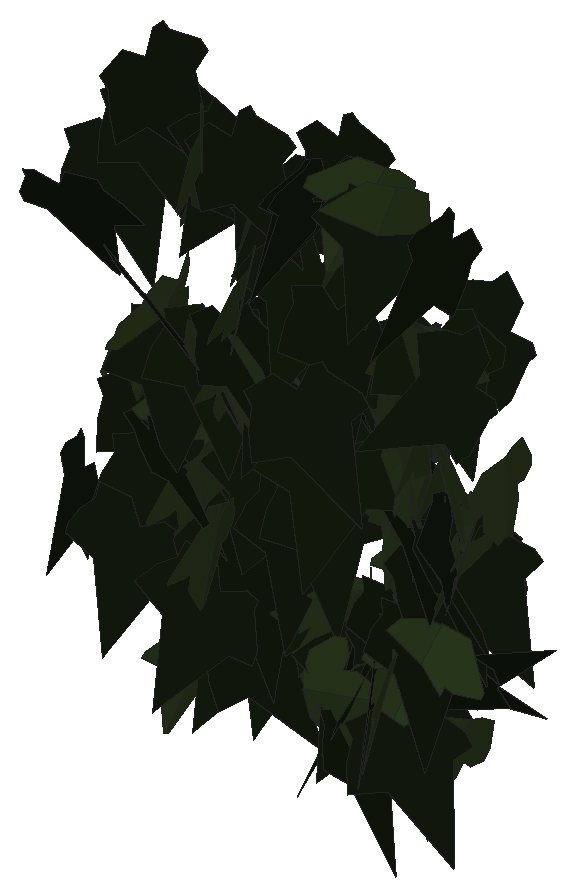
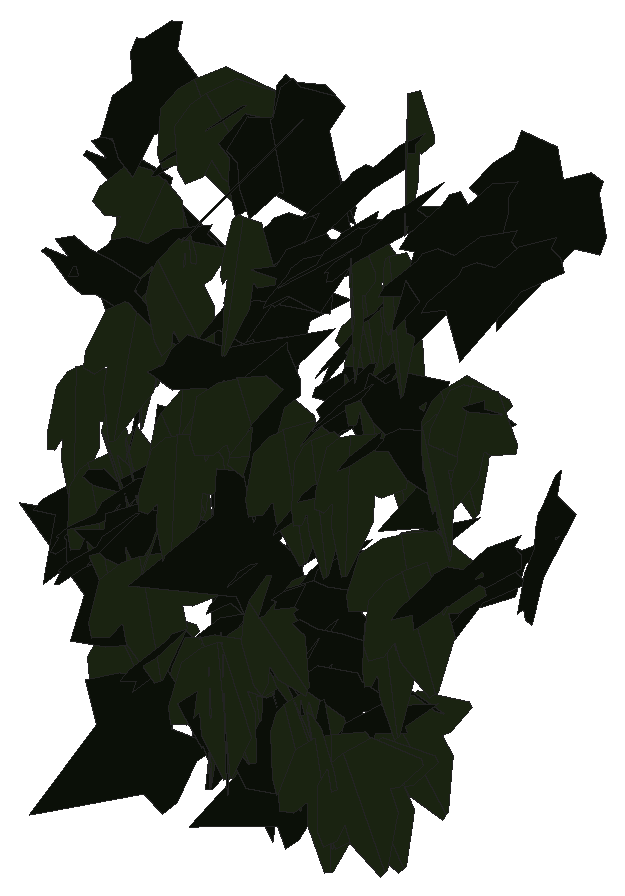
# SketchUp Ruby script. Lengths in inches.
U = 1.inch
M = Sketchup.active_model
def pt(a) = Geom::Point3d.new(a.map { |v| v * U })
def face(e, loops, mat)
  f = e.add_face(loops[0].map { |a| pt(a) })
  loops[1..].each { |l| e.add_face(l.map { |a| pt(a) }).erase! }
  f.material = f.back_material = mat if mat
  f
end
# faces: each face lists its corners as indices into pts; further lists are holes
def faces(e, pts, list, mat = nil) = list.each { |f| face(e, (f[0].is_a?(Array) ? f : [f]).map { |l| l.map { |i| pts[i] } }, mat) }
# xy, xz, yz: faces in a plane at the given z, y or x. An outline is a flat list of corners, or four numbers for a rectangle; further outlines are holes
def ring(l) = l.size == 4 ? [[l[0], l[1]], [l[2], l[1]], [l[2], l[3]], [l[0], l[3]]] : l.each_slice(2).to_a
def flat(e, list, mat, &to3) = list.each { |f| face(e, (f[0].is_a?(Array) ? f : [f]).map { |l| ring(l).map { |u, v| to3.(u, v) } }, mat) }
def xy(e, z, list, mat = nil) = flat(e, list, mat) { |x, y| [x, y, z] }
def xz(e, y, list, mat = nil) = flat(e, list, mat) { |x, z| [x, y, z] }
def yz(e, x, list, mat = nil) = flat(e, list, mat) { |y, z| [x, y, z] }
def lines(e, pts, list) = list.each { |a, b| e.add_line(pt(pts[a]), pt(pts[b])) }
# prism: a flat outline (further loops are holes) pulled along v
def prism(e, loops, v, mat = nil)
  f = face(e, loops, mat); d = Geom::Vector3d.new(v.map { |x| x * U })
  f.pushpull(f.normal.samedirection?(d) ? d.length : -d.length)
end
def box(e, o, s, mat = nil) = prism(e, [[o, [o[0] + s[0], o[1], o[2]], [o[0] + s[0], o[1] + s[1], o[2]], [o[0], o[1] + s[1], o[2]]]], [0, 0, s[2]], mat)
def at(x, y, z, deg = 0) = Geom::Transformation.translation(pt([x, y, z])) * Geom::Transformation.rotation(ORIGIN, Z_AXIS, deg.degrees)
def axes(o, x, y, z) = Geom::Transformation.new([*x, 0, *y, 0, *z, 0, *pt(o).to_a, 1])
def part(name) = M.definitions.add(name)
# library, detail: a bought-in or finely detailed component or shape, given as its bounding box
def library(name, o, s) = part(name).tap { |d| box(d.entities, o, s) }
def detail(e, o, s) = box(e.add_group.entities, o, s)
def put(e, d, t, mat = nil) = e.add_instance(d, t).tap { |i| i.material = mat if mat }
def group(e, t, mat = nil) = e.add_group.tap { |g| g.transformation = t; g.material = mat if mat }.entities
root = M.entities
M.materials.add("efeu1").color = [18, 25, 13]
M.materials.add("efeu2").color = [43, 57, 29]
c1 = part("ivyleaf_9")
p = [[1.54,2.16,1.25],[1.36,2.04,1.19],[-0.21,0.99,0.68],[-0.71,1.11,0.82],[-0.85,0.86,0.67],[-0.8,0.17,0.21],
  [-0.9,-0.01,0.1],[-0.67,-0.16,-0.02],[-0.08,-0.08,-0.05],[-0.03,-0.6,-0.4],[0.65,-0.88,-0.66],[0.83,-0.6,-0.49],
  [1.29,-0.42,-0.43],[1.8125,-0.07,-0.26],[1.21,0.44,0.15]]
faces(c1.entities,p,[[0,1,2,3,4,5,6,7,8,9,10,11,12,13,14]],"efeu1")
c2 = part("ivyleaf_10")
p = [[0,0.5,-0.03],[-0.0625,2.02,-0.43],[-0.19,2.01,-0.46],[-0.54,1.05,-0.29],[-0.52,0.625,-0.18],[-0.83,0.76,-0.28],
  [-1.16,0.64,-0.33],[-1.15,0.33,-0.24],[-0.77,-0.39,0.02],[-0.3,-0.51,0.16],[0.04,-0.48,0.23],[-0.02,2.01,-0.4375],
  [-0.06,2.01,-0.43],[0.04,-0.49,0.23],[0.67,-0.49,0.14],[1.38,0.36,-0.2],[1.375,0.51,-0.24],[0.81,0.65,-0.19],
  [0.62,0.59,-0.15],[0.6,1.09,-0.28],[0.5,1.23,-0.31]]
faces(c2.entities,p,[[0,1,2,3,4,5,6,7,8,9,10],[11,12,0,13,14,15,16,17,18,19,20]],"efeu2")
put(root,c1,axes([21.94,221.7,247.83],[-0.00718,-0.45611,-0.20472],[0.00835,0.2046,-0.45615],[0.49988,-0.00997,0.00468]))
put(root,c1,axes([21.98,222.09,248.62],[0.12472,-0.32873,-0.35551],[-0.11519,0.33643,-0.35149],[0.47029,0.16958,0.00819]))
put(root,c1,axes([21.98,222.13,244.82],[0.06592,-0.45564,-0.19506],[-0.00933,0.1956,-0.46006],[0.49555,0.06429,0.01728]))
put(root,c1,axes([22.02,222.2,248.14],[-0.002,-0.44065,-0.23628],[0.02599,0.23587,-0.4401],[0.49932,-0.01404,0.02196]))
put(root,c2,axes([22.24,222.24,246.03],[0.20254,-0.45532,-0.04074],[-0.00639,0.04173,-0.49821],[0.4571,0.20233,0.01109]))
put(root,c1,axes([22.11,220.87,244.48],[0.0514,-0.1225,-0.48203],[0.39843,-0.2799,0.11362],[-0.29768,-0.39579,0.06885]))
put(root,c1,axes([22.26,220.36,248.03],[0.43986,0.19109,-0.14144],[-0.12527,-0.06654,-0.47946],[-0.20207,0.45723,-0.01067]))
put(root,c2,axes([22.37,221.54,246.09],[-0.05994,-0.43878,-0.23212],[0.06327,0.22515,-0.44193],[0.49235,-0.08235,0.02853]))
put(root,c2,axes([22.43,222.34,244.48],[-0.20804,-0.43866,0.11957],[0.00303,-0.13282,-0.48203],[0.45465,-0.19984,0.05793]))
put(root,c2,axes([22.47,221.68,246.08],[-0.01427,-0.49342,0.07959],[0.00788,-0.07984,-0.49352],[0.49973,-0.01283,0.01005]))
put(root,c2,axes([22.53,222.3,244.82],[-0.35573,-0.34113,0.08416],[0.01746,-0.13678,-0.48061],[0.35093,-0.339,0.10922]))
put(root,c2,axes([22.67,222.24,247.66],[0.13927,-0.44991,-0.16789],[-0.04136,0.16292,-0.4709],[0.47843,0.14505,0.00817]))
put(root,c1,axes([22.47,221.78,244.32],[-0.09242,-0.47478,-0.12667],[0.04032,0.12113,-0.48343],[0.48973,-0.09957,0.0159]))
put(root,c2,axes([22.8125,222.1875,243.95],[0.04057,-0.49503,-0.05741],[0.00034,0.05762,-0.49667],[0.49835,0.04026,0.00501]))
put(root,c1,axes([22.7,221.02,243.94],[-0.10273,-0.46976,0.13699],[0.00798,-0.14157,-0.47947],[0.48927,-0.09633,0.03658]))
put(root,c1,axes([22.72,221.72,245.86],[-0.14691,-0.46907,-0.09159],[0.03101,0.08626,-0.49153],[0.47692,-0.1501,0.00375]))
put(root,c2,axes([22.93,222.54,242.49],[-0.10601,-0.47011,0.13326],[-0.00024,-0.13631,-0.48106],[0.48863,-0.10206,0.02867]))
put(root,c2,axes([22.92,221.68,244.43],[-0.0495,-0.47632,-0.14378],[0.03239,0.1411,-0.47858],[0.49649,-0.05669,0.01688]))
put(root,c2,axes([22.99,222.29,242.35],[-0.13086,-0.44973,0.17498],[-0.01304,-0.17794,-0.46709],[0.48239,-0.12681,0.03484]))
put(root,c2,axes([23.04,222.43,245.72],[-0.05034,-0.47661,-0.14251],[0.0096,0.14228,-0.47923],[0.49737,-0.05098,-0.00517]))
put(root,c2,axes([23.06,221.63,242.52],[-0.08309,-0.44521,0.21185],[0.00959,-0.21626,-0.45071],[0.49295,-0.07084,0.04448]))
put(root,c2,axes([23.19,222.53,242.5625],[-0.22687,-0.44358,-0.04205],[0.02165,0.03615,-0.49822],[0.44504,-0.22788,0.0028]))
put(root,c1,axes([22.86,221.06,245.08],[0.3603,-0.34484,0.0357],[0.03065,-0.0196,-0.49867],[0.34532,0.36153,0.00701]))
put(root,c1,axes([23.11,222.16,247.91],[-0.15095,-0.40278,0.25491],[-0.02749,-0.25959,-0.42645],[0.47588,-0.14276,0.05622]))
put(root,c2,axes([23.3125,222.59,245.65],[0.03476,-0.49595,-0.05316],[0.00722,0.05379,-0.49705],[0.49874,0.03379,0.0109]))
put(root,c1,axes([23.27,222.25,242.69],[-0.23801,-0.4244,0.11505],[-0.0315,-0.11403,-0.4858],[0.43859,-0.2385,0.02754]))
put(root,c1,axes([23.14,222.59,245.61],[0.04574,-0.49787,-0.00559],[-0.00178,0.00545,-0.49997],[0.4979,0.04575,-0.00127]))
put(root,c2,axes([23.36,222.54,242.77],[0.33224,-0.35276,-0.12319],[-0.04442,0.12638,-0.48172],[0.371,0.33104,0.05264]))
put(root,c1,axes([23.25,221.66,246.13],[-0.24943,-0.34197,-0.26616],[0.18372,0.19468,-0.42231],[0.39247,-0.30847,0.02854]))
put(root,c2,axes([23.41,221.08,248.6],[0.19754,-0.42153,-0.18247],[0.00708,0.2014,-0.45759],[0.45927,0.1782,0.08554]))
put(root,c2,axes([23.43,221.9,247.39],[0.22939,-0.42739,-0.12134],[0.01425,0.14356,-0.47874],[0.44405,0.21617,0.07804]))
put(root,c1,axes([23.09,220.61,247],[0.16255,-0.31502,0.35262],[0.24397,-0.26354,-0.34789],[0.40504,0.28516,0.06803]))
put(root,c1,axes([23.5,222.36,244.3],[-0.21717,-0.42753,0.14161],[-0.02373,-0.14614,-0.47758],[0.44975,-0.21415,0.04319]))
put(root,c1,axes([23.4375,221.72,246.11],[0.24836,-0.17624,-0.39655],[-0.16607,0.38353,-0.27446],[0.40092,0.26804,0.13197]))
put(root,c2,axes([23.64,222.6,245.65],[-0.14138,-0.47872,0.02891],[-0.0035,-0.02911,-0.49914],[0.47958,-0.14134,0.00488]))
put(root,c2,axes([23.56,221.2,246.28],[-0.4763,0.11152,-0.10346],[0.09587,-0.04398,-0.48875],[-0.11811,-0.48542,0.02051]))
put(root,c1,axes([23.89,222.0625,243.34],[-0.46642,-0.0595,0.17002],[-0.16454,-0.05133,-0.46935],[0.07331,-0.49379,0.0283]))
put(root,c1,axes([23.45,222.3,247.73],[-0.00126,-0.49882,-0.03433],[-0.00018,0.03433,-0.49882],[0.5,-0.00124,-0.00027]))
put(root,c2,axes([23.64,221.47,246.125],[0.07402,-0.49395,-0.02322],[-0.00096,0.02333,-0.49945],[0.49449,0.07398,0.00251]))
put(root,c1,axes([23.52,222.3,247.61],[-0.12755,-0.45786,0.15523],[0.0016,-0.16094,-0.47339],[0.48345,-0.12027,0.04253]))
put(root,c1,axes([23.4,221.7,248.37],[0.17978,-0.4135,-0.2161],[-0.01419,0.22664,-0.44546],[0.46635,0.1663,0.06976]))
put(root,c1,axes([23.83,222.33,243.92],[-0.40993,-0.27045,0.09391],[-0.06187,-0.07644,-0.49023],[0.27952,-0.41354,0.02921]))
put(root,c2,axes([23.75,222.39,242.64],[0.05964,-0.49612,0.01766],[-0.00553,-0.01845,-0.49963],[0.4964,0.0594,-0.00769]))
put(root,c2,axes([23.85,221.25,247.09],[0.14322,-0.4684,-0.10045],[-0.02757,0.09661,-0.4898],[0.47826,0.14584,0.00184]))
put(root,c1,axes([23.71,222.18,245.67],[-0.10409,-0.43227,0.22871],[-0.00969,-0.23196,-0.44283],[0.48895,-0.09662,0.03991]))
put(root,c2,axes([23.81,222.75,243.94],[0.07966,-0.42983,0.24269],[0.05337,-0.23689,-0.43707],[0.49072,0.09554,0.00814]))
put(root,c1,axes([23.8,222.11,243.07],[-0.36458,-0.29719,-0.16958],[0.16858,0.05964,-0.46693],[0.29776,-0.39765,0.05671]))
put(root,c1,axes([23.68,221.72,243.61],[0.10279,-0.48695,0.04808],[0.00492,-0.0481,-0.49766],[0.48929,0.10279,-0.00509]))
put(root,c1,axes([23.88,220.8125,243.7],[-0.20317,-0.42789,0.16012],[-0.03606,-0.15967,-0.47245],[0.45544,-0.20352,0.03402]))
put(root,c1,axes([23.75,221.23,246.52],[0.2045,-0.44623,-0.09519],[-0.02707,0.09226,-0.49067],[0.45546,0.20584,0.01358]))
put(root,c1,axes([23.65,222.31,242.27],[0.46922,-0.13208,0.11131],[0.10724,-0.02983,-0.48745],[0.13541,0.48132,0.00034]))
put(root,c1,axes([23.79,221.35,243],[0.21128,-0.36279,-0.27156],[-0.0483,0.2799,-0.41149],[0.45059,0.20011,0.08323]))
put(root,c1,axes([23.87,222.18,244],[-0.01863,-0.49061,0.09465],[-0.00595,-0.09449,-0.49096],[0.49962,-0.01942,-0.00232]))
put(root,c1,axes([24.1,222.28,244.25],[0.00324,-0.49504,-0.07017],[0.00903,0.07021,-0.49496],[0.49991,0.00194,0.00939]))
put(root,c2,axes([24.31,220.21,244.84],[0.05786,-0.49376,-0.05345],[-0.00545,0.05318,-0.49713],[0.49661,0.05812,0.00077]))
put(root,c2,axes([24.25,222.03,242.8],[0.40826,-0.28855,-0.00756],[-0.00851,0.00104,-0.49993],[0.28853,0.40833,-0.00406]))
put(root,c2,axes([24.41,222.13,243.15],[-0.22378,-0.41359,0.1699],[-0.08715,-0.146,-0.4702],[0.43855,-0.24005,-0.00675]))
put(root,c1,axes([24.53,222.11,242.74],[0.24869,0.14386,-0.40922],[-0.38698,-0.13952,-0.28422],[-0.19596,0.45808,0.04194]))
put(root,c1,axes([24.3,221.91,247.13],[-0.21059,-0.45266,0.02746],[-0.00304,-0.02886,-0.49916],[0.45348,-0.2104,0.0094]))
put(root,c2,axes([24.51,222.21,245.72],[-0.43822,-0.16536,0.175],[-0.12714,-0.14969,-0.45981],[0.20446,-0.44749,0.08915]))
put(root,c1,axes([24.01,222.38,244.55],[0.45017,-0.02172,0.21652],[0.21744,0.02545,-0.44953],[0.00851,0.49888,0.03236]))
put(root,c2,axes([24.41,221.67,245.03],[0.09092,-0.19493,0.45137],[-0.14135,0.42928,0.21386],[-0.47091,-0.16649,0.02295]))
put(root,c2,axes([24.41,222.3125,247.5],[0.06951,-0.41177,-0.27498],[0.00253,0.27797,-0.4156],[0.49514,0.05639,0.04073]))
put(root,c1,axes([24.55,221.87,245.96],[0.25961,0.13789,-0.40446],[-0.42339,0.01895,-0.2653],[-0.05784,0.48024,0.1266]))
put(root,c2,axes([24.5,222.53,243.07],[-0.23539,-0.44086,0.01524],[-0.00544,-0.01437,-0.49976],[0.44109,-0.23544,0.00197]))
put(root,c1,axes([24.71,222.26,242.86],[-0.03675,0.10075,-0.48836],[-0.47739,0.13436,0.06364],[0.14405,0.47095,0.08632]))
put(root,c1,axes([24.6,221.6,248.39],[-0.06855,0.29064,-0.40103],[0.11306,-0.38498,-0.29834],[-0.4822,-0.13158,-0.01294]))
put(root,c1,axes([24.26,222.33,248.38],[0.24287,-0.42199,-0.11375],[-0.00206,0.12903,-0.48306],[0.43705,0.23511,0.06094]))
put(root,c1,axes([24.61,221.59,248.4],[-0.12475,0.24861,-0.41549],[0.17865,-0.37515,-0.27811],[-0.45002,-0.21785,0.00477]))
put(root,c2,axes([24.67,222.42,243.08],[0.46403,-0.00277,-0.18619],[-0.18209,0.09791,-0.45526],[0.03898,0.49031,0.08985]))
put(root,c1,axes([25.04,221.99,245.67],[-0.07232,0.197,0.45383],[-0.49418,-0.05069,-0.05675],[0.02365,-0.45675,0.20204]))
put(root,c1,axes([24.75,221.99,242.21],[-0.0227,-0.02223,0.49899],[0.16778,0.47014,0.02858],[-0.47046,0.16874,-0.01388]))
put(root,c2,axes([24.79,222.31,242.84],[0.21144,-0.39774,-0.21702],[-0.04211,0.2212,-0.44643],[0.45113,0.20706,0.06004]))
put(root,c1,axes([24.65,221.8,246.75],[0.04484,-0.49712,-0.02941],[-0.00572,0.02901,-0.49912],[0.49795,0.04509,-0.00308]))
put(root,c2,axes([24.93,221.96,242.61],[-0.01534,-0.48953,0.10064],[-0.00012,-0.10068,-0.48976],[0.49976,-0.01505,0.00297]))
put(root,c2,axes([24.59,222.04,242.31],[-0.03961,0.0065,-0.49839],[0.3893,-0.3118,-0.035],[-0.31125,-0.39081,0.01964]))
put(root,c2,axes([25.08,221.83,248.39],[-0.26564,-0.34996,0.23866],[-0.06802,-0.24282,-0.43176],[0.4181,-0.26185,0.08139]))
put(root,c1,axes([24.92,222.02,242.68],[-0.1881,-0.42817,0.17688],[0.00958,-0.19446,-0.46054],[0.46317,-0.16986,0.08136]))
put(root,c2,axes([25.08,222.43,245.01],[-0.0714,-0.48105,-0.11616],[0.03648,0.11192,-0.48594],[0.49353,-0.07786,0.01911]))
put(root,c2,axes([25.33,221.74,245.27],[0.2958,-0.23407,-0.3282],[-0.24936,0.21361,-0.37708],[0.31674,0.38676,0.00964]))
put(root,c2,axes([25.21,222.78,243.85],[-0.31125,-0.3802,0.09257],[0.01722,-0.13147,-0.4821],[0.39093,-0.29692,0.09493]))
put(root,c1,axes([25.27,221.4375,243.03],[-0.34118,0.20476,-0.30277],[0.23697,-0.19141,-0.39649],[-0.27828,-0.41405,0.03357]))
put(root,c1,axes([24.98,222.44,243.09],[0.04027,-0.47399,0.15398],[0.05989,-0.14876,-0.47359],[0.49476,0.05658,0.04479]))
put(root,c1,axes([24.95,222.79,242.4],[0.46641,0.11333,0.14006],[0.12064,0.09226,-0.47638],[-0.13382,0.47817,0.05871]))
put(root,c1,axes([25.03,222.3,243.09],[0.12335,-0.38562,-0.2934],[-0.02848,0.29647,-0.40162],[0.48371,0.11579,0.05117]))
put(root,c2,axes([24.86,221.31,242.75],[0.11192,-0.04526,-0.48521],[0.443,-0.19797,0.12065],[-0.20303,-0.4569,-0.00421]))
put(root,c2,axes([25.39,221.67,248.34],[-0.24851,-0.40195,0.16335],[-0.03191,-0.17081,-0.46883],[0.4327,-0.24344,0.05925]))
put(root,c2,axes([25.18,221.89,245.58],[-0.36009,0.28831,-0.1929],[0.16258,-0.10535,-0.46094],[-0.30643,-0.39469,-0.01787]))
put(root,c1,axes([25.17,221.45,242.21],[0.21354,-0.44862,0.05604],[0.01611,-0.05439,-0.49677],[0.45182,0.21397,-0.00878]))
put(root,c2,axes([25.47,222.03,246.6],[0.04716,-0.46713,0.17194],[0.0068,-0.17209,-0.4694],[0.49772,0.04661,-0.00988]))
put(root,c1,axes([25.39,220.91,245.82],[-0.21717,-0.44959,-0.02656],[0.00803,0.02562,-0.49928],[0.4503,-0.21728,-0.00391]))
put(root,c1,axes([25.34,221.76,248.06],[-0.14051,-0.45123,0.16326],[0.02854,-0.17767,-0.4665],[0.479,-0.12177,0.07569]))
put(root,c2,axes([25.43,222.28,244.33],[-0.2854,0.40742,-0.05055],[0.03438,-0.03763,-0.4974],[-0.4091,-0.28739,-0.00654]))
put(root,c1,axes([25.25,220.44,246.65],[0.09525,-0.44066,-0.21621],[0.05478,0.22841,-0.4414],[0.48778,0.0604,0.09179]))
put(root,c2,axes([25.52,221.95,244.95],[0.05701,-0.45688,0.19495],[0.07544,-0.18599,-0.45795],[0.49098,0.08163,0.04772]))
put(root,c1,axes([25.75,222.6,244.14],[-0.36242,-0.33961,0.05756],[-0.04613,-0.03494,-0.49664],[0.34135,-0.3653,-0.00601]))
put(root,c1,axes([25.51,222.07,242.55],[0.00986,-0.49938,-0.0229],[0.00143,0.02293,-0.49947],[0.4999,0.00978,0.00188]))
put(root,c2,axes([25.71,222.28,246.125],[-0.15871,-0.44656,-0.15937],[0.06156,0.14723,-0.47385],[0.47013,-0.17003,0.00824]))
put(root,c2,axes([25.9,222,243.68],[0.177,-0.46473,-0.0519],[-0.01578,0.04953,-0.49729],[0.46736,0.17768,0.00286]))
put(root,c1,axes([25.83,222.64,243.98],[-0.15748,-0.43287,0.19448],[0.00172,-0.20542,-0.45585],[0.47455,-0.14291,0.06619]))
put(root,c1,axes([25.65,221.82,244.48],[0.09079,-0.32401,0.36983],[0.12685,-0.34792,-0.33595],[0.47504,0.15483,0.01902]))
put(root,c1,axes([26.22,222.52,246.79],[-0.49313,0.00694,0.08229],[-0.08218,0.00796,-0.49314],[-0.00815,-0.49989,-0.00671]))
put(root,c1,axes([25.87,222.61,244.3],[-0.14528,-0.44946,0.16395],[0.00169,-0.17182,-0.46955],[0.47843,-0.13588,0.05144]))
put(root,c2,axes([26.06,221.5,246.9],[-0.47285,0.14529,0.07283],[-0.09382,-0.06106,-0.48731],[-0.13271,-0.47451,0.08501]))
put(root,c1,axes([25.76,221.03,243.48],[-0.06557,-0.06536,-0.49135],[0.45669,-0.20065,-0.03425],[-0.19271,-0.45328,0.08601]))
put(root,c1,axes([25.82,221.97,246.84],[-0.06196,-0.44695,-0.2154],[0.09686,0.202,-0.44701],[0.4866,-0.09712,0.06156]))
put(root,c1,axes([25.79,222.17,244.3],[0.19232,-0.45944,0.0439],[0.01749,-0.04026,-0.49807],[0.4612,0.19312,0.00059]))
put(root,c2,axes([26.09,222.375,244.35],[0.00863,-0.49967,-0.01606],[-0.0035,0.016,-0.49973],[0.49991,0.00874,-0.00322]))
put(root,c2,axes([26.11,221.35,246.17],[0.10734,-0.40832,-0.26786],[-0.0485,0.26399,-0.42185],[0.48593,0.11655,0.01707]))
put(root,c2,axes([26.03,222.18,244.67],[0.31107,-0.38979,0.03606],[0.01803,-0.03174,-0.49867],[0.39104,0.31154,-0.00569]))
put(root,c2,axes([26.16,221.84,242.43],[-0.12321,-0.45412,0.16909],[-0.05424,-0.16045,-0.47044],[0.48154,-0.13426,-0.00972]))
put(root,c2,axes([26.11,221.75,244.34],[0.22948,-0.43715,-0.07896],[-0.03757,0.06946,-0.49373],[0.44264,0.23253,-0.00097]))
put(root,c1,axes([25.88,221.65,244.42],[0.26847,-0.37055,-0.20152],[-0.06581,0.19916,-0.45388],[0.41664,0.27023,0.05817]))
put(root,c2,axes([26.18,221.57,245.8],[0.1397,-0.41472,-0.24184],[-0.05538,0.23627,-0.43716],[0.47688,0.14893,0.02008]))
put(root,c2,axes([26.09,221.58,247.03],[-0.47695,0.10904,-0.1031],[0.10182,-0.01717,-0.48922],[-0.11023,-0.48766,-0.00582]))
put(root,c1,axes([26.06,222.14,244.31],[0.01209,-0.37725,-0.32792],[0.05508,0.32703,-0.37419],[0.49681,-0.02707,0.04946]))
put(root,c1,axes([26.25,221.58,248.24],[-0.08087,0.01673,-0.49313],[0.27874,-0.41079,-0.05965],[-0.40714,-0.28456,0.05711]))
put(root,c2,axes([26.3,221.41,245.88],[-0.39838,0.30118,0.02424],[-0.02113,0.01224,-0.4994],[-0.30141,-0.39893,0.00298]))
put(root,c2,axes([26.3,222.37,245.27],[0.00664,-0.49179,-0.08997],[0.05222,0.09017,-0.48902],[0.49722,-0.00291,0.05256]))
put(root,c1,axes([25.97,221.66,243.0625],[0.30854,0.32795,-0.21737],[0.15166,0.15575,0.45027],[0.36304,-0.34379,-0.00336]))
put(root,c1,axes([26.2,221.62,244.82],[-0.01575,-0.06537,0.49546],[-0.01994,-0.49523,-0.06598],[0.49935,-0.02183,0.013]))
put(root,c2,axes([26.33,220.45,243.79],[0.29681,-0.38095,0.12952],[0.07933,-0.10238,-0.48293],[0.39447,0.30723,-0.00034]))
put(root,c2,axes([26.45,221.01,243.92],[0.38485,0.251,-0.19721],[-0.16486,-0.10823,-0.45946],[-0.27334,0.41867,-0.00054]))
put(root,c1,axes([26.25,221.15,243.87],[0.05036,-0.4832,0.11826],[0.03419,-0.11522,-0.48534],[0.49628,0.05697,0.02144]))
put(root,c1,axes([26.86,221.15,246.99],[-0.48331,0.05206,0.11705],[-0.11596,0.01638,-0.48609],[-0.05445,-0.49701,-0.00376]))
put(root,c1,axes([26.37,220.69,243.07],[0.04622,-0.44691,-0.21939],[0.05258,0.22348,-0.44417],[0.49507,0.01798,0.06766]))
